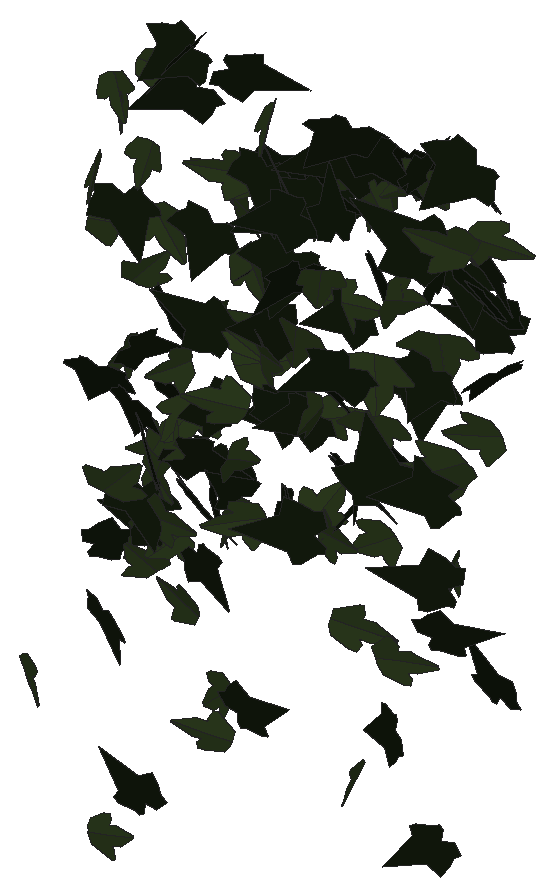
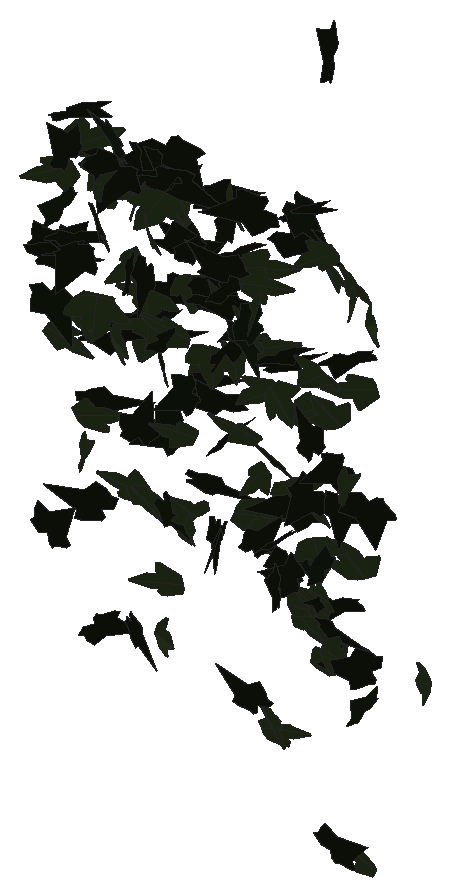
# SketchUp Ruby script. Lengths in inches.
U = 1.inch
M = Sketchup.active_model
def pt(a) = Geom::Point3d.new(a.map { |v| v * U })
def face(e, loops, mat)
  f = e.add_face(loops[0].map { |a| pt(a) })
  loops[1..].each { |l| e.add_face(l.map { |a| pt(a) }).erase! }
  f.material = f.back_material = mat if mat
  f
end
# faces: each face lists its corners as indices into pts; further lists are holes
def faces(e, pts, list, mat = nil) = list.each { |f| face(e, (f[0].is_a?(Array) ? f : [f]).map { |l| l.map { |i| pts[i] } }, mat) }
# xy, xz, yz: faces in a plane at the given z, y or x. An outline is a flat list of corners, or four numbers for a rectangle; further outlines are holes
def ring(l) = l.size == 4 ? [[l[0], l[1]], [l[2], l[1]], [l[2], l[3]], [l[0], l[3]]] : l.each_slice(2).to_a
def flat(e, list, mat, &to3) = list.each { |f| face(e, (f[0].is_a?(Array) ? f : [f]).map { |l| ring(l).map { |u, v| to3.(u, v) } }, mat) }
def xy(e, z, list, mat = nil) = flat(e, list, mat) { |x, y| [x, y, z] }
def xz(e, y, list, mat = nil) = flat(e, list, mat) { |x, z| [x, y, z] }
def yz(e, x, list, mat = nil) = flat(e, list, mat) { |y, z| [x, y, z] }
def lines(e, pts, list) = list.each { |a, b| e.add_line(pt(pts[a]), pt(pts[b])) }
# prism: a flat outline (further loops are holes) pulled along v
def prism(e, loops, v, mat = nil)
  f = face(e, loops, mat); d = Geom::Vector3d.new(v.map { |x| x * U })
  f.pushpull(f.normal.samedirection?(d) ? d.length : -d.length)
end
def box(e, o, s, mat = nil) = prism(e, [[o, [o[0] + s[0], o[1], o[2]], [o[0] + s[0], o[1] + s[1], o[2]], [o[0], o[1] + s[1], o[2]]]], [0, 0, s[2]], mat)
def at(x, y, z, deg = 0) = Geom::Transformation.translation(pt([x, y, z])) * Geom::Transformation.rotation(ORIGIN, Z_AXIS, deg.degrees)
def axes(o, x, y, z) = Geom::Transformation.new([*x, 0, *y, 0, *z, 0, *pt(o).to_a, 1])
def part(name) = M.definitions.add(name)
# library, detail: a bought-in or finely detailed component or shape, given as its bounding box
def library(name, o, s) = part(name).tap { |d| box(d.entities, o, s) }
def detail(e, o, s) = box(e.add_group.entities, o, s)
def put(e, d, t, mat = nil) = e.add_instance(d, t).tap { |i| i.material = mat if mat }
def group(e, t, mat = nil) = e.add_group.tap { |g| g.transformation = t; g.material = mat if mat }.entities
root = M.entities
M.materials.add("1026 AP 7946 SUNNY SIDE UP").color = [254, 231, 186]
M.materials.add("efeu1").color = [18, 25, 13]
M.materials.add("efeu2").color = [43, 57, 29]
c1 = part("ivyleaf_9")
p = [[1.54,2.16,1.25],[1.36,2.04,1.19],[-0.21,0.99,0.68],[-0.71,1.11,0.82],[-0.85,0.86,0.67],[-0.8,0.17,0.21],
  [-0.9,-0.01,0.1],[-0.67,-0.16,-0.02],[-0.08,-0.08,-0.05],[-0.03,-0.6,-0.4],[0.65,-0.88,-0.66],[0.83,-0.6,-0.49],
  [1.29,-0.42,-0.43],[1.8125,-0.07,-0.26],[1.21,0.44,0.15]]
faces(c1.entities,p,[[0,1,2,3,4,5,6,7,8,9,10,11,12,13,14]],"efeu1")
c2 = part("ivyleaf_10")
p = [[0,0.5,-0.03],[-0.0625,2.02,-0.43],[-0.19,2.01,-0.46],[-0.54,1.05,-0.29],[-0.52,0.625,-0.18],[-0.83,0.76,-0.28],
  [-1.16,0.64,-0.33],[-1.15,0.33,-0.24],[-0.77,-0.39,0.02],[-0.3,-0.51,0.16],[0.04,-0.48,0.23],[-0.02,2.01,-0.4375],
  [-0.06,2.01,-0.43],[0.04,-0.49,0.23],[0.67,-0.49,0.14],[1.38,0.36,-0.2],[1.375,0.51,-0.24],[0.81,0.65,-0.19],
  [0.62,0.59,-0.15],[0.6,1.09,-0.28],[0.5,1.23,-0.31]]
faces(c2.entities,p,[[0,1,2,3,4,5,6,7,8,9,10],[11,12,0,13,14,15,16,17,18,19,20]],"efeu2")
put(root,c1,axes([126.25,209.5,261.4],[0.31609,0.13219,-0.20378],[-0.24736,-0.12173,-0.24827],[-0.28195,0.25499,-0.01064]),"1026 AP 7946 SUNNY SIDE UP")
put(root,c1,axes([125.875,209.98,257.64],[0.13575,0.07095,0.30954],[0.4401,0.11269,-0.10975],[-0.2034,0.29119,-0.03089]),"1026 AP 7946 SUNNY SIDE UP")
put(root,c2,axes([126.11,207.73,256.31],[-0.17013,0.16637,-0.26384],[0.18273,-0.22991,-0.20504],[-0.44543,-0.15786,0.01665]),"1026 AP 7946 SUNNY SIDE UP")
put(root,c1,axes([126.17,209.77,256.47],[0.10924,-0.27762,0.17798],[0.05098,-0.17152,-0.29569],[0.51293,0.07617,-0.00852]),"1026 AP 7946 SUNNY SIDE UP")
put(root,c2,axes([126.31,209.98,266.57],[-0.13345,0.19894,-0.23402],[0.09498,-0.2212,-0.223],[-0.46656,-0.10193,0.02154]),"1026 AP 7946 SUNNY SIDE UP")
put(root,c1,axes([126.84,210,252.9375],[0.0317,-0.00398,0.3272],[-0.34147,0.23211,0.01855],[-0.36454,-0.21777,0.01107]),"1026 AP 7946 SUNNY SIDE UP")
put(root,c2,axes([126.33,209.85,266.88],[0.36723,-0.06966,0.19975],[0.27917,-0.08182,-0.25056],[0.1655,0.29257,-0.02057]),"1026 AP 7946 SUNNY SIDE UP")
put(root,c2,axes([126.24,209.63,264.27],[-0.04544,-0.05543,-0.35241],[0.48576,0.15072,-0.05121],[0.24581,-0.30809,0.03606]),"1026 AP 7946 SUNNY SIDE UP")
put(root,c2,axes([126.6,210.43,258.07],[0.02789,-0.23251,0.23617],[0.04013,-0.22922,-0.2415],[0.51332,0.03055,0.00605]),"1026 AP 7946 SUNNY SIDE UP")
put(root,c2,axes([126.43,209.22,265.56],[0.1737,-0.13033,0.30198],[0.25034,-0.24777,-0.1763],[0.43914,0.1928,-0.01894]),"1026 AP 7946 SUNNY SIDE UP")
put(root,c1,axes([127,210.1,258.38],[-0.22725,-0.05078,-0.26104],[-0.38537,-0.06412,0.15705],[-0.1275,0.28432,-0.0094]),"1026 AP 7946 SUNNY SIDE UP")
put(root,c2,axes([126.68,209.875,261.77],[-0.00258,0.00437,-0.34384],[-0.08107,-0.32979,-0.00611],[-0.5186,0.05153,0.00267]),"1026 AP 7946 SUNNY SIDE UP")
put(root,c2,axes([126.39,209.36,252.43],[0.14227,-0.08564,-0.27123],[0.37469,-0.11593,0.12276],[-0.2202,-0.2526,0.03366]),"1026 AP 7946 SUNNY SIDE UP")
put(root,c2,axes([126.93,210.12,257.49],[-0.25104,-0.15023,-0.1946],[-0.233,-0.11647,0.22478],[-0.29823,0.21745,-0.01181]),"1026 AP 7946 SUNNY SIDE UP")
put(root,c1,axes([126.74,209.6,264.87],[-0.11121,-0.32192,-0.12384],[0.05785,0.11305,-0.3387],[0.53622,-0.07896,0.01086]),"1026 AP 7946 SUNNY SIDE UP")
put(root,c2,axes([126.81,209.16,259.43],[-0.40043,-0.14281,0.16554],[0.2022,0.09998,0.30057],[-0.27207,0.28449,-0.02025]),"1026 AP 7946 SUNNY SIDE UP")
put(root,c1,axes([126.84,209.98,259.02],[-0.20731,-0.26733,-0.15684],[0.12753,0.12786,-0.30597],[0.46541,-0.15412,0.01398]),"1026 AP 7946 SUNNY SIDE UP")
put(root,c1,axes([127.07,209.43,261.06],[0.35855,-0.00451,-0.22458],[-0.3421,-0.02499,-0.23409],[-0.02205,0.31446,-0.01997]),"1026 AP 7946 SUNNY SIDE UP")
put(root,c2,axes([126.96,209.78,263.33],[-0.22121,-0.21747,0.1607],[0.1118,0.14097,0.26723],[-0.40687,0.15697,-0.01394]),"1026 AP 7946 SUNNY SIDE UP")
put(root,c1,axes([126.99,209.54,262.06],[0.01595,0.10057,-0.29313],[-0.06877,0.28276,0.1028],[0.47038,0.03793,0.02497]),"1026 AP 7946 SUNNY SIDE UP")
put(root,c2,axes([126.82,210.27,259.2],[0.13786,0.0012,0.28347],[0.40129,-0.10831,-0.08392],[0.16174,0.2677,-0.03341]),"1026 AP 7946 SUNNY SIDE UP")
put(root,c1,axes([126.92,210.24,259.86],[0.2093,-0.21589,0.17952],[0.11474,-0.16063,-0.26155],[0.42215,0.1507,-0.01792]),"1026 AP 7946 SUNNY SIDE UP")
put(root,c2,axes([127.02,209.97,267.43],[0.11786,0.10905,0.29432],[0.18937,0.25916,-0.13324],[-0.44099,0.14043,0.02144]),"1026 AP 7946 SUNNY SIDE UP")
put(root,c2,axes([127.41,209.875,260.11],[-0.34645,-0.25507,0.055],[-0.02904,-0.05635,-0.34678],[0.40921,-0.21995,0.02195]),"1026 AP 7946 SUNNY SIDE UP")
put(root,c2,axes([127.51,210.05,258.3],[0.40311,-0.05283,-0.14651],[-0.22837,-0.00684,-0.26771],[0.06736,0.29294,-0.0309]),"1026 AP 7946 SUNNY SIDE UP")
put(root,c2,axes([127.14,210.01,264.45],[0.42493,0.03457,0.24637],[0.37811,-0.00633,-0.27926],[-0.0341,0.36068,-0.02639]),"1026 AP 7946 SUNNY SIDE UP")
put(root,c2,axes([127.22,209.9,258.62],[-0.13724,0.03101,0.33158],[0.50524,-0.02731,0.09236],[0.05435,0.33219,-0.02139]),"1026 AP 7946 SUNNY SIDE UP")
put(root,c1,axes([127.35,210.05,262.61],[-0.01017,-0.05653,0.34656],[0.16694,-0.32042,-0.05519],[0.51026,0.1037,0.02496]),"1026 AP 7946 SUNNY SIDE UP")
put(root,c1,axes([127.58,209.79,261.35],[0.4913,-0.04058,-0.09505],[-0.14887,-0.01723,-0.3234],[0.05341,0.32527,-0.02705]),"1026 AP 7946 SUNNY SIDE UP")
put(root,c2,axes([127.77,208.96,266.43],[0.42477,-0.18086,0.06258],[0.05759,-0.05599,-0.33419],[0.29494,0.2714,-0.02488]),"1026 AP 7946 SUNNY SIDE UP")
put(root,c1,axes([128.12,209.77,267.43],[0.0397,0.00778,-0.34628],[-0.25272,-0.29584,-0.02122],[-0.46443,0.16165,-0.01805]),"1026 AP 7946 SUNNY SIDE UP")
put(root,c1,axes([127.98,209.86,268.08],[-0.32587,-0.21029,0.21606],[-0.17032,-0.18614,-0.30193],[0.43626,-0.22976,0.04351]),"1026 AP 7946 SUNNY SIDE UP")
put(root,c2,axes([127.7,209.36,260.49],[0.41134,-0.14577,-0.06258],[0.10498,-0.00268,0.30699],[-0.22449,-0.26836,0.02889]),"1026 AP 7946 SUNNY SIDE UP")
put(root,c1,axes([128.02,209.75,268.16],[-0.25588,0.24847,-0.22682],[0.16246,-0.19677,-0.30663],[-0.49764,-0.19199,0.01653]),"1026 AP 7946 SUNNY SIDE UP")
put(root,c2,axes([128.23,209.62,261.22],[0.4013,0.13943,-0.18251],[-0.22025,-0.11313,-0.29893],[-0.27902,0.28983,-0.02653]),"1026 AP 7946 SUNNY SIDE UP")
put(root,c1,axes([127.85,210.03,259.23],[0.30233,-0.19542,0.15894],[0.15157,-0.12282,-0.28271],[0.36215,0.21455,-0.01436]),"1026 AP 7946 SUNNY SIDE UP")
put(root,c1,axes([128.24,210.12,264.62],[-0.24068,-0.3065,0.06039],[-0.02074,-0.06081,-0.35295],[0.49076,-0.15288,0.0147]),"1026 AP 7946 SUNNY SIDE UP")
put(root,c1,axes([128.03,210.41,259.13],[0.04352,-0.03299,-0.34177],[0.48919,-0.11658,0.03802],[-0.18761,-0.31163,0.01986]),"1026 AP 7946 SUNNY SIDE UP")
put(root,c1,axes([128.19,210.26,260.15],[-0.00558,-0.28717,0.0074],[0.00245,-0.00883,-0.29591],[0.45176,-0.0035,0.0017]),"1026 AP 7946 SUNNY SIDE UP")
put(root,c2,axes([128.7,208.92,257.81],[-0.11868,0.03911,-0.30519],[-0.37957,0.17251,0.08777],[0.27754,0.25265,-0.01048]),"1026 AP 7946 SUNNY SIDE UP")
put(root,c2,axes([128.55,210.0625,255.66],[0.27523,-0.21079,-0.17935],[-0.19194,0.12313,-0.28123],[0.38331,0.21301,-0.01204]),"1026 AP 7946 SUNNY SIDE UP")
put(root,c2,axes([128.62,208.89,262.57],[0.05594,0.0174,-0.34687],[-0.24747,-0.29868,-0.03476],[-0.46901,0.15967,-0.02303]),"1026 AP 7946 SUNNY SIDE UP")
put(root,c2,axes([128.8,209.64,255.03],[0.06559,0.05937,0.29509],[-0.37845,-0.1569,0.06877],[0.26054,-0.24286,0.02561]),"1026 AP 7946 SUNNY SIDE UP")
put(root,c2,axes([128.63,209.7,263.3],[-0.05193,-0.35345,0.13217],[-0.00967,-0.13028,-0.36642],[0.59225,-0.03312,0.00561]),"1026 AP 7946 SUNNY SIDE UP")
put(root,c1,axes([128.25,209.32,260.57],[0.08481,0.03694,-0.32267],[0.25403,0.26991,0.06299],[0.42628,-0.16819,0.02666]),"1026 AP 7946 SUNNY SIDE UP")
put(root,c1,axes([129.06,209.46,261.6],[-0.41164,0.2492,0.09515],[-0.14708,0.03285,-0.36992],[-0.39032,-0.27518,0.03905]),"1026 AP 7946 SUNNY SIDE UP")
put(root,c2,axes([129.16,209.89,265.96],[-0.04263,-0.02234,-0.34281],[-0.52304,-0.02051,0.02923],[-0.03506,0.33311,-0.01923]),"1026 AP 7946 SUNNY SIDE UP")
put(root,c1,axes([128.93,210.04,259.63],[0.06637,0.06015,0.30272],[-0.363,-0.1824,0.07164],[0.30028,-0.23379,0.01969]),"1026 AP 7946 SUNNY SIDE UP")
put(root,c2,axes([129.27,209.67,266.2],[-0.00967,-0.03677,-0.36987],[-0.5119,-0.15395,0.0211],[-0.2442,0.32418,-0.02958]),"1026 AP 7946 SUNNY SIDE UP")
put(root,c2,axes([129.02,209.88,265.48],[-0.14625,0.21461,0.24705],[-0.18218,0.20919,-0.23916],[-0.47056,-0.14769,0.01581]),"1026 AP 7946 SUNNY SIDE UP")
put(root,c1,axes([129.32,208.95,263.47],[-0.26413,-0.27952,-0.10689],[-0.09268,-0.08375,0.33539],[-0.45869,0.17788,-0.00621]),"1026 AP 7946 SUNNY SIDE UP")
put(root,c1,axes([128.83,209.04,258.83],[-0.0905,-0.04554,-0.31006],[0.47376,0.03321,-0.0644],[0.06523,-0.30437,0.03753]),"1026 AP 7946 SUNNY SIDE UP")
put(root,c1,axes([128.82,209.99,267.92],[0.13892,0.06423,-0.3334],[0.18661,0.30682,0.09779],[0.48469,-0.13654,0.05791]),"1026 AP 7946 SUNNY SIDE UP")
put(root,c1,axes([128.9375,210.04,265.14],[0.44051,-0.18907,-0.01186],[-0.03258,-0.01208,-0.34755],[0.29596,0.28009,-0.02061]),"1026 AP 7946 SUNNY SIDE UP")
put(root,c2,axes([128.94,209.44,263.21],[0.24573,0.18215,0.27617],[0.31261,0.17971,-0.2451],[-0.40077,0.25187,-0.02185]),"1026 AP 7946 SUNNY SIDE UP")
put(root,c2,axes([129.27,209.62,259.66],[0.07165,-0.26815,0.20436],[0.06732,-0.19541,-0.28124],[0.52158,0.06205,0.00823]),"1026 AP 7946 SUNNY SIDE UP")
put(root,c1,axes([129.51,209.74,264.51],[-0.11869,0.30491,0.09218],[-0.0448,0.08332,-0.32302],[-0.49688,-0.08035,0.0071]),"1026 AP 7946 SUNNY SIDE UP")
put(root,c2,axes([129.43,209.2,260.9],[-0.06992,-0.15121,-0.29319],[0.15756,0.26566,-0.16047],[0.48037,-0.10914,0.00996]),"1026 AP 7946 SUNNY SIDE UP")
put(root,c1,axes([129.17,209.74,255.6],[-0.00383,0.03701,0.31039],[0.34882,-0.20515,0.02663],[0.32534,0.22039,-0.0249]),"1026 AP 7946 SUNNY SIDE UP")
put(root,c2,axes([129.12,210.02,262.27],[0.26647,-0.09976,-0.2861],[0.4617,0.0319,0.17333],[-0.03667,-0.32328,0.1033]),"1026 AP 7946 SUNNY SIDE UP")
put(root,c2,axes([129.85,209.25,259.8125],[0.14196,0.03233,-0.34396],[-0.42024,-0.20233,-0.09576],[-0.31922,0.28074,-0.02689]),"1026 AP 7946 SUNNY SIDE UP")
put(root,c2,axes([129.375,209.65,264.57],[0.34195,-0.05758,0.31815],[0.44877,-0.12167,-0.23089],[0.20761,0.35786,-0.02492]),"1026 AP 7946 SUNNY SIDE UP")
put(root,c1,axes([129.81,210.11,259.74],[0.18766,-0.148,-0.26879],[-0.3007,0.17763,-0.19351],[0.3619,0.22434,-0.0214]),"1026 AP 7946 SUNNY SIDE UP")
put(root,c1,axes([129.97,210.09,259.79],[0.22221,-0.0628,-0.29227],[-0.4247,0.08686,-0.1581],[0.16698,0.30449,-0.01318]),"1026 AP 7946 SUNNY SIDE UP")
put(root,c1,axes([129.76,209.72,266.4375],[-0.13316,-0.34214,0.00887],[0.01143,-0.01267,-0.36303],[0.53812,-0.0844,0.00991]),"1026 AP 7946 SUNNY SIDE UP")
put(root,c1,axes([129.92,209.93,265.6],[0.05527,-0.1626,-0.31428],[0.12148,-0.29423,0.16953],[-0.5285,-0.08464,0.0061]),"1026 AP 7946 SUNNY SIDE UP")
put(root,c1,axes([129.66,210.08,266.1],[-0.12462,0.0377,0.30448],[0.45364,-0.06582,0.08802],[0.11572,0.29862,-0.01718]),"1026 AP 7946 SUNNY SIDE UP")
put(root,c2,axes([129.79,209.75,267.54],[0.26886,-0.18966,0.26553],[0.22438,-0.21774,-0.26276],[0.45191,0.22095,-0.02751]),"1026 AP 7946 SUNNY SIDE UP")
put(root,c1,axes([130.03,209.85,261.72],[0.1103,-0.25039,-0.22435],[0.1281,-0.20129,0.26602],[-0.50432,-0.10589,0.0185]),"1026 AP 7946 SUNNY SIDE UP")
put(root,c1,axes([130.27,209.59,263.5],[-0.15131,-0.07389,0.36813],[-0.36876,-0.27116,-0.12427],[0.44041,-0.25243,0.02242]),"1026 AP 7946 SUNNY SIDE UP")
put(root,c1,axes([130.1875,209.36,266.86],[0.36958,-0.12756,-0.1952],[-0.28189,0.06377,-0.27401],[0.22103,0.29463,-0.02307]),"1026 AP 7946 SUNNY SIDE UP")
put(root,c2,axes([130.55,207.83,262.91],[0.03705,0.1205,0.33052],[-0.2495,-0.28044,0.11914],[0.47651,-0.15621,0.03668]),"1026 AP 7946 SUNNY SIDE UP")
put(root,c1,axes([130.41,209.61,265.01],[-0.41302,-0.26975,-0.05491],[0.08782,0.01768,-0.38674],[0.42287,-0.26714,0.02669]),"1026 AP 7946 SUNNY SIDE UP")
put(root,c2,axes([130.13,209.15,263.14],[-0.21437,0.06131,0.33603],[0.44685,-0.15986,0.15255],[0.26854,0.31496,0.0144]),"1026 AP 7946 SUNNY SIDE UP")
put(root,c2,axes([130.56,209.57,263.56],[-0.53994,0.0049,0.06689],[-0.1023,-0.03584,-0.35203],[0.00294,-0.34762,0.03518]),"1026 AP 7946 SUNNY SIDE UP")
put(root,c1,axes([130.57,209.13,262.09],[-0.29356,0.0088,0.26241],[0.39854,0.03902,0.19026],[-0.04139,0.31335,-0.0292]),"1026 AP 7946 SUNNY SIDE UP")
put(root,c2,axes([130.61,210.05,259.86],[0.25516,0.17014,-0.23041],[0.21107,0.18124,0.24238],[0.38958,-0.20963,0.0196]),"1026 AP 7946 SUNNY SIDE UP")
put(root,c1,axes([131.21,209.11,260.05],[-0.42669,0.0474,0.22778],[-0.35119,-0.00489,-0.28168],[-0.05291,-0.34983,0.03272]),"1026 AP 7946 SUNNY SIDE UP")
put(root,c1,axes([130.93,209.13,265.1],[-0.08513,0.1877,-0.32193],[0.08865,-0.3089,-0.20233],[-0.56775,-0.07638,0.01668]),"1026 AP 7946 SUNNY SIDE UP")
put(root,c1,axes([131.02,209.72,266.06],[-0.48948,-0.0122,0.23043],[0.34572,0.05729,0.31868],[-0.06801,0.37906,-0.03847]),"1026 AP 7946 SUNNY SIDE UP")
put(root,c1,axes([131.19,210.26,260],[-0.25863,0.23733,-0.13589],[0.09916,-0.11823,-0.29781],[-0.41633,-0.17559,0.01349]),"1026 AP 7946 SUNNY SIDE UP")
put(root,c2,axes([130.7,210.13,259.44],[-0.12003,0.05553,0.34095],[0.50391,-0.08757,0.09086],[0.15493,0.32785,-0.03137]),"1026 AP 7946 SUNNY SIDE UP")
put(root,c1,axes([130.71,209.97,266.24],[0.14682,-0.08795,0.29206],[0.26556,-0.22929,-0.13169],[0.38473,0.19183,-0.02055]),"1026 AP 7946 SUNNY SIDE UP")
put(root,c2,axes([130.75,210.1,261.76],[0.13991,-0.00107,-0.29117],[0.41405,0.10797,0.08561],[0.16147,-0.27594,0.03277]),"1026 AP 7946 SUNNY SIDE UP")
put(root,c1,axes([130.88,209.82,262.63],[0.44043,-0.13519,0.00735],[-0.00555,-0.02544,-0.31956],[0.21286,0.27905,-0.02354]),"1026 AP 7946 SUNNY SIDE UP")
put(root,c2,axes([131.23,209.36,265],[-0.343,-0.2312,0.01505],[0.01051,-0.02814,-0.32668],[0.36425,-0.2169,0.0236]),"1026 AP 7946 SUNNY SIDE UP")
put(root,c1,axes([131.34,209.07,262.44],[-0.01462,-0.15018,-0.29017],[-0.028,-0.28024,0.15337],[-0.49994,0.02009,-0.00011]),"1026 AP 7946 SUNNY SIDE UP")
put(root,c1,axes([131.36,210.22,263.95],[0.02075,-0.19017,-0.27296],[0.02007,-0.26359,0.19482],[-0.51106,-0.01808,-0.00343]),"1026 AP 7946 SUNNY SIDE UP")
put(root,c1,axes([131.45,208.44,266.68],[-0.06744,-0.16827,-0.30899],[-0.01544,-0.30058,0.17397],[-0.53924,0.02965,0.03366]),"1026 AP 7946 SUNNY SIDE UP")
put(root,c2,axes([131.37,209.46,266.59],[0.25604,-0.32293,0.15461],[0.08639,-0.14231,-0.37314],[0.55447,0.17129,-0.01326]),"1026 AP 7946 SUNNY SIDE UP")
put(root,c2,axes([131,210.09,264.13],[0.10039,-0.09057,-0.34076],[0.51751,-0.07662,0.08674],[-0.14881,-0.32754,0.07177]),"1026 AP 7946 SUNNY SIDE UP")
put(root,c1,axes([131.83,209.63,267.46],[-0.01209,-0.0605,-0.4143],[-0.35948,-0.3316,0.054],[-0.52822,0.22706,-0.02727]),"1026 AP 7946 SUNNY SIDE UP")
put(root,c2,axes([131.4375,208.96,262.61],[0.00236,-0.01285,0.35201],[0.19093,-0.31948,-0.01479],[0.50274,0.12139,0.00397]),"1026 AP 7946 SUNNY SIDE UP")
put(root,c2,axes([131.23,210,257.93],[0.04587,0.05484,0.3307],[0.40237,0.19498,-0.05719],[-0.31593,0.25628,-0.02482]),"1026 AP 7946 SUNNY SIDE UP")
put(root,c1,axes([131.87,209.36,268.09],[0.15655,0.16973,-0.32918],[-0.21528,-0.29017,-0.20382],[-0.52806,0.16862,-0.0145]),"1026 AP 7946 SUNNY SIDE UP")
put(root,c2,axes([131.65,210.24,266.47],[0.30016,-0.18534,0.19856],[0.20902,-0.14119,-0.27483],[0.36619,0.23251,-0.00588]),"1026 AP 7946 SUNNY SIDE UP")
put(root,c2,axes([132.06,210.07,259.87],[0.35555,-0.09875,-0.21398],[-0.3052,0.07283,-0.25362],[0.19249,0.29788,-0.00689]),"1026 AP 7946 SUNNY SIDE UP")
put(root,c2,axes([131.75,209.78,267.02],[-0.43384,-0.21046,-0.17845],[0.25085,0.07308,-0.35528],[0.34605,-0.31682,0.03382]),"1026 AP 7946 SUNNY SIDE UP")
put(root,c1,axes([131.55,209.52,261.36],[0.49316,-0.16452,0.05283],[0.04985,-0.05155,-0.3638],[0.26679,0.31375,-0.02968]),"1026 AP 7946 SUNNY SIDE UP")
put(root,c1,axes([131.91,210.29,261.45],[0.37185,-0.19834,0.09053],[-0.07758,0.07911,0.31714],[-0.33292,-0.23997,0.02721]),"1026 AP 7946 SUNNY SIDE UP")
put(root,c1,axes([132.1,209.82,265.22],[0.35808,-0.10041,-0.2719],[-0.40713,0.05923,-0.25357],[0.17509,0.34309,-0.03356]),"1026 AP 7946 SUNNY SIDE UP")
put(root,c1,axes([132.19,208.55,266.64],[-0.21969,-0.19095,0.27823],[0.20285,0.23977,0.24383],[-0.48041,0.18857,-0.02428]),"1026 AP 7946 SUNNY SIDE UP")
put(root,c1,axes([132.49,209.77,256.375],[-0.00093,-0.01296,-0.34917],[-0.52807,0.04704,-0.00098],[0.07398,0.33559,-0.01134]),"1026 AP 7946 SUNNY SIDE UP")
put(root,c2,axes([132.32,209.83,266.73],[-0.07594,0.3594,-0.13799],[-0.04577,0.13324,0.37421],[0.60249,0.05542,0.01104]),"1026 AP 7946 SUNNY SIDE UP")
put(root,c1,axes([132.55,208.41,264.09],[0.0356,-0.00003,-0.36464],[-0.24621,-0.31808,-0.01215],[-0.49914,0.1569,-0.02001]),"1026 AP 7946 SUNNY SIDE UP")
put(root,c2,axes([132.29,209.0625,255.85],[0.14588,-0.20349,0.22334],[0.11349,-0.20615,-0.23113],[0.45492,0.11668,-0.01396]),"1026 AP 7946 SUNNY SIDE UP")
put(root,c1,axes([131.95,209.56,267.75],[-0.00328,-0.04866,-0.36922],[0.48048,0.19101,-0.02746],[0.30347,-0.30294,0.03948]),"1026 AP 7946 SUNNY SIDE UP")
put(root,c1,axes([132.1,210.35,265.33],[0.10595,-0.07824,-0.32501],[0.43812,-0.15113,0.09918],[-0.26187,-0.28451,0.03444]),"1026 AP 7946 SUNNY SIDE UP")
put(root,c2,axes([132.55,210.26,263.54],[0.21229,-0.25945,0.20453],[0.12809,-0.18294,-0.3022],[0.49893,0.15736,-0.00944]),"1026 AP 7946 SUNNY SIDE UP")
put(root,c2,axes([132.88,210.2,267.14],[-0.07868,-0.11832,0.34329],[-0.16048,-0.3181,-0.13374],[0.5334,-0.11316,0.0104]),"1026 AP 7946 SUNNY SIDE UP")
put(root,c1,axes([132.6875,210.02,267.58],[0.52027,0.096,-0.12543],[-0.16803,-0.06847,-0.3536],[-0.17758,0.34605,-0.03291]),"1026 AP 7946 SUNNY SIDE UP")
put(root,c2,axes([132.73,209.43,265.07],[-0.04657,-0.16392,-0.36236],[0.21846,0.32391,-0.1661],[0.56832,-0.13794,0.03416]),"1026 AP 7946 SUNNY SIDE UP")
put(root,c2,axes([132.91,208.75,263],[-0.53284,-0.11613,-0.02214],[0.04786,-0.02482,-0.36758],[0.17923,-0.3386,0.03232]),"1026 AP 7946 SUNNY SIDE UP")
put(root,c2,axes([132.73,208.9,263.98],[0.58945,0.08156,0.07224],[0.11926,-0.02252,-0.39347],[-0.11926,0.38063,-0.03642]),"1026 AP 7946 SUNNY SIDE UP")
put(root,c1,axes([132.8,208.49,262.37],[-0.2033,0.01712,-0.36705],[0.50321,-0.16206,-0.12857],[-0.24809,-0.34274,0.04]),"1026 AP 7946 SUNNY SIDE UP")
put(root,c1,axes([133.03,209.96,263.38],[-0.27762,-0.30506,-0.08089],[0.08193,0.05848,-0.36242],[0.48781,-0.18343,0.01484]),"1026 AP 7946 SUNNY SIDE UP")
put(root,c2,axes([133.42,210.1875,261.34],[0.1313,0.09426,0.31106],[-0.37589,-0.18486,0.1267],[0.32449,-0.25228,0.02091]),"1026 AP 7946 SUNNY SIDE UP")
put(root,c2,axes([133.23,210.14,264.07],[-0.55256,-0.19201,-0.0203],[0.05309,-0.02314,-0.41096],[0.29864,-0.35114,0.0355]),"1026 AP 7946 SUNNY SIDE UP")
put(root,c1,axes([133.24,209.875,263.59],[-0.23634,-0.28255,0.088],[-0.03712,-0.08584,-0.32964],[0.4634,-0.15098,0.01847]),"1026 AP 7946 SUNNY SIDE UP")
put(root,c2,axes([133.21,209.79,267.41],[-0.35682,-0.19044,-0.12605],[0.16861,0.06041,-0.30407],[0.31242,-0.25011,0.02014]),"1026 AP 7946 SUNNY SIDE UP")
put(root,c1,axes([133.26,209.28,267.62],[-0.12474,0.32112,0.08672],[0.0303,-0.08007,0.34029],[0.52039,0.08164,0.00098]),"1026 AP 7946 SUNNY SIDE UP")
put(root,c1,axes([133.65,209.45,265.59],[0.00413,0.11702,0.33214],[-0.01348,0.32167,-0.11858],[-0.53817,-0.00716,0.00552]),"1026 AP 7946 SUNNY SIDE UP")
put(root,c1,axes([134.11,208.75,266.72],[-0.50562,-0.17419,-0.20627],[-0.29684,-0.06874,0.3754],[-0.29162,0.37198,-0.02449]),"1026 AP 7946 SUNNY SIDE UP")
put(root,c1,axes([133.81,207.83,262.43],[-0.4519,-0.21451,0.21824],[0.23654,0.15354,0.36918],[-0.41238,0.32314,-0.0274]),"1026 AP 7946 SUNNY SIDE UP")
put(root,c1,axes([133.73,210.125,265.34],[0.55044,0.00356,-0.16567],[-0.25073,-0.04336,-0.35878],[-0.03351,0.3828,-0.03683]),"1026 AP 7946 SUNNY SIDE UP")
put(root,c2,axes([133.46,208.41,258.7],[-0.15124,0.00386,0.31967],[0.45164,0.12403,0.09086],[-0.18463,0.30024,-0.03959]),"1026 AP 7946 SUNNY SIDE UP")
put(root,c1,axes([133.74,210.22,265.68],[-0.21887,-0.284,-0.11374],[0.10192,0.08919,-0.32478],[0.46722,-0.15249,0.01757]),"1026 AP 7946 SUNNY SIDE UP")
put(root,c2,axes([133.87,209.77,260.07],[0.00246,0.05628,-0.33559],[-0.00837,-0.32603,-0.0599],[-0.52023,0.00551,-0.00062]),"1026 AP 7946 SUNNY SIDE UP")
put(root,c1,axes([133.61,209.52,258.73],[0.09434,0.01811,0.31445],[0.48014,-0.01757,-0.06089],[0.02166,0.31048,-0.01996]),"1026 AP 7946 SUNNY SIDE UP")
put(root,c1,axes([134.32,210.12,264.99],[0.29692,-0.07271,0.30732],[-0.40479,0.15426,0.20723],[-0.26428,-0.31796,0.02787]),"1026 AP 7946 SUNNY SIDE UP")
put(root,c1,axes([133.73,201.4,266.22],[0.18799,-0.11634,-0.44396],[0.62961,-0.16769,0.16034],[-0.30793,-0.41391,0.05682]),"1026 AP 7946 SUNNY SIDE UP")
put(root,c1,axes([134.29,208.75,255.3],[-0.00314,-0.06941,-0.32097],[0.02356,-0.31085,0.06952],[-0.50075,-0.01419,0.00528]),"1026 AP 7946 SUNNY SIDE UP")
put(root,c2,axes([134.53,209.82,262.84],[0.23448,-0.05858,-0.30819],[-0.45612,0.07391,-0.16362],[0.14568,0.32569,-0.01624]),"1026 AP 7946 SUNNY SIDE UP")
put(root,c1,axes([133.92,210.1875,267.55],[0.10676,-0.19579,0.31951],[0.16178,-0.29376,-0.2152],[0.5551,0.12327,0.00127]),"1026 AP 7946 SUNNY SIDE UP")
put(root,c1,axes([134.63,208.5,260.49],[-0.23243,-0.00008,0.32078],[-0.47904,-0.0712,-0.14943],[0.10119,-0.33725,0.02941]),"1026 AP 7946 SUNNY SIDE UP")
put(root,c1,axes([134.68,210.11,264.77],[-0.20845,0.05357,0.31583],[-0.48818,-0.00483,-0.1376],[-0.0264,-0.3337,0.05069]),"1026 AP 7946 SUNNY SIDE UP")
put(root,c1,axes([134.46,210.08,263.91],[-0.05037,0.34961,-0.09322],[0.00317,-0.09267,-0.36215],[-0.56862,-0.03149,0.00624]),"1026 AP 7946 SUNNY SIDE UP")
put(root,c1,axes([134.4,209.55,268.1875],[-0.38724,-0.26255,0.17414],[-0.14184,-0.14826,-0.37022],[0.47139,-0.26029,0.03166]),"1026 AP 7946 SUNNY SIDE UP")
put(root,c2,axes([134.72,208.77,266.98],[-0.18472,-0.10744,-0.36165],[-0.48157,-0.1734,0.15952],[-0.31664,0.3264,-0.03164]),"1026 AP 7946 SUNNY SIDE UP")
put(root,c1,axes([134.67,208.44,262.34],[-0.29776,-0.09445,0.32932],[-0.40577,-0.19213,-0.21673],[0.33303,-0.31855,0.03037]),"1026 AP 7946 SUNNY SIDE UP")
put(root,c2,axes([134.74,208.6,262.88],[-0.28898,-0.11335,0.32469],[-0.38233,-0.20316,-0.22207],[0.3636,-0.30372,0.02455]),"1026 AP 7946 SUNNY SIDE UP")
put(root,c1,axes([134.17,210.1,266.12],[0.21149,-0.31228,0.12932],[0.05894,-0.12237,-0.35074],[0.52698,0.13901,-0.01267]),"1026 AP 7946 SUNNY SIDE UP")
put(root,c1,axes([134.75,209.82,257.87],[0.18828,-0.14363,0.29067],[-0.23375,0.24181,0.19267],[-0.44083,-0.18956,0.02198]),"1026 AP 7946 SUNNY SIDE UP")
put(root,c2,axes([134.49,209.63,266.77],[-0.15093,-0.11509,-0.33605],[0.45763,0.15487,-0.1439],[0.29217,-0.30202,0.05178]),"1026 AP 7946 SUNNY SIDE UP")
